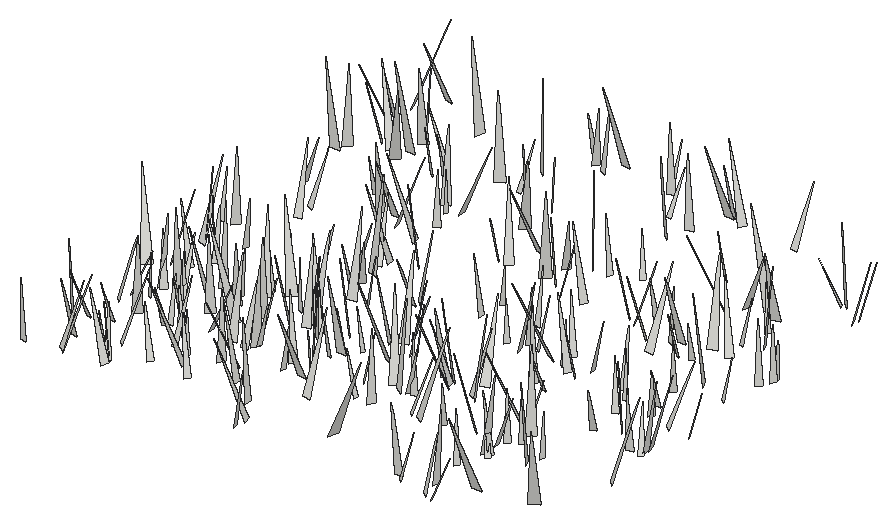
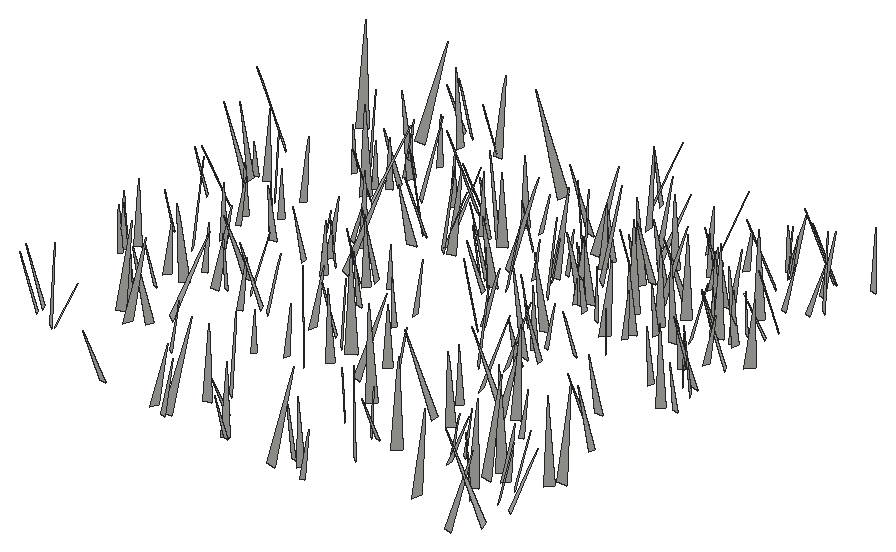
# SketchUp Ruby script. Lengths in inches.
U = 1.inch
M = Sketchup.active_model
def pt(a) = Geom::Point3d.new(a.map { |v| v * U })
def face(e, loops, mat)
  f = e.add_face(loops[0].map { |a| pt(a) })
  loops[1..].each { |l| e.add_face(l.map { |a| pt(a) }).erase! }
  f.material = f.back_material = mat if mat
  f
end
# faces: each face lists its corners as indices into pts; further lists are holes
def faces(e, pts, list, mat = nil) = list.each { |f| face(e, (f[0].is_a?(Array) ? f : [f]).map { |l| l.map { |i| pts[i] } }, mat) }
# xy, xz, yz: faces in a plane at the given z, y or x. An outline is a flat list of corners, or four numbers for a rectangle; further outlines are holes
def ring(l) = l.size == 4 ? [[l[0], l[1]], [l[2], l[1]], [l[2], l[3]], [l[0], l[3]]] : l.each_slice(2).to_a
def flat(e, list, mat, &to3) = list.each { |f| face(e, (f[0].is_a?(Array) ? f : [f]).map { |l| ring(l).map { |u, v| to3.(u, v) } }, mat) }
def xy(e, z, list, mat = nil) = flat(e, list, mat) { |x, y| [x, y, z] }
def xz(e, y, list, mat = nil) = flat(e, list, mat) { |x, z| [x, y, z] }
def yz(e, x, list, mat = nil) = flat(e, list, mat) { |y, z| [x, y, z] }
def lines(e, pts, list) = list.each { |a, b| e.add_line(pt(pts[a]), pt(pts[b])) }
# prism: a flat outline (further loops are holes) pulled along v
def prism(e, loops, v, mat = nil)
  f = face(e, loops, mat); d = Geom::Vector3d.new(v.map { |x| x * U })
  f.pushpull(f.normal.samedirection?(d) ? d.length : -d.length)
end
def box(e, o, s, mat = nil) = prism(e, [[o, [o[0] + s[0], o[1], o[2]], [o[0] + s[0], o[1] + s[1], o[2]], [o[0], o[1] + s[1], o[2]]]], [0, 0, s[2]], mat)
def at(x, y, z, deg = 0) = Geom::Transformation.translation(pt([x, y, z])) * Geom::Transformation.rotation(ORIGIN, Z_AXIS, deg.degrees)
def axes(o, x, y, z) = Geom::Transformation.new([*x, 0, *y, 0, *z, 0, *pt(o).to_a, 1])
def part(name) = M.definitions.add(name)
# library, detail: a bought-in or finely detailed component or shape, given as its bounding box
def library(name, o, s) = part(name).tap { |d| box(d.entities, o, s) }
def detail(e, o, s) = box(e.add_group.entities, o, s)
def put(e, d, t, mat = nil) = e.add_instance(d, t).tap { |i| i.material = mat if mat }
def group(e, t, mat = nil) = e.add_group.tap { |g| g.transformation = t; g.material = mat if mat }.entities
root = M.entities
c1 = part("fur_instance\#9")
p = [[0.8125,0,1.79],[0.67,-0.02,1.48],[0,-0.11,0],[0,0.11,0]]
faces(c1.entities,p,[[0,1,2,3]])
put(root,c1,axes([495.33,166.6,-21.66],[4.4988,1.24272,1.44893],[1.33102,-4.70119,-0.10058],[-1.36826,-0.48722,4.6662]))
put(root,c1,axes([455.36,167.15,-21.66],[1.09401,4.63876,2.44173],[5.21296,-1.22556,-0.00737],[-0.55243,-2.37843,4.76601]))
put(root,c1,axes([531.0625,167.53,-21.66],[3.86213,1.08614,0.2172],[1.09096,-3.86634,-0.0646],[-0.19154,-0.12107,4.01143]))
put(root,c1,axes([495.47,169.01,-21.66],[-6.50715,-2.26194,0.29712],[-2.26712,6.51165,-0.07913],[0.25462,0.17236,6.88863]))
put(root,c1,axes([529.4375,167.89,-21.66],[2.64561,4.33348,1.24236],[4.47199,-2.70465,-0.08904],[-0.56902,-1.10798,5.07645]))
put(root,c1,axes([522.83,170.07,-21.66],[0.27233,-6.25887,1.87066],[-6.53155,-0.29195,-0.02597],[-0.1084,1.8677,6.26474]))
put(root,c1,axes([469.08,168.99,-21.66],[-5.48361,2.04542,0.49712],[2.0602,5.49974,0.09665],[0.43181,-0.2646,5.85187]))
put(root,c1,axes([524,169,-21.66],[2.95956,2.83712,0.75066],[2.89518,-2.997,-0.08741],[-0.48027,-0.58351,4.09885]))
put(root,c1,axes([461.68,168.53,-21.66],[4.96936,4.425,0.65774],[4.44372,-4.99597,0.03757],[-0.51632,-0.4092,6.65385]))
put(root,c1,axes([461.31,168.68,-21.66],[3.13584,4.70476,0.63652],[4.72939,-3.16238,0.0748],[-0.41563,-0.48786,5.65355]))
put(root,c1,axes([534.39,173.77,-21.66],[-0.28609,-7.90952,0.17476],[-7.91116,0.28452,-0.07401],[-0.06767,0.17732,7.91434]))
put(root,c1,axes([468.52,170.24,-21.66],[-1.71851,4.03919,1.0736],[4.16688,1.74577,0.10182],[0.32374,-1.02868,4.3884]))
put(root,c1,axes([467.48,171.24,-21.66],[-3.40834,-0.81843,0.94444],[-0.85751,3.5273,-0.03792],[0.90911,0.25869,3.50503]))
put(root,c1,axes([528.77,171.32,-21.66],[6.1687,-0.67373,2.21616],[-0.70194,-6.55164,-0.0379],[-2.20738,0.2006,6.20527]))
put(root,c1,axes([467.7,171.68,-21.66],[-3.21218,-2.63282,1.4726],[-2.81239,3.39173,-0.07071],[1.09119,0.99138,4.15269]))
put(root,c1,axes([460.17,173,-21.66],[-1.26664,-5.03308,1.07763],[-5.14261,1.28411,-0.04714],[0.2163,1.05675,5.1898]))
put(root,c1,axes([507.95,173.49,-21.66],[8.10386,-2.02713,0.06413],[-2.02706,-8.10412,-0.01624],[-0.06615,-0.00019,8.35354]))
put(root,c1,axes([492.31,173.19,-21.66],[-6.58404,0.20466,2.39247],[0.20033,7.00521,-0.04793],[2.39284,-0.02336,6.58705]))
put(root,c1,axes([543.59,175.66,-21.66],[4.25947,-6.86655,0.67935],[-6.89421,-4.26807,0.08653],[-0.2843,0.62304,8.07992]))
put(root,c1,axes([481,173.25,-21.66],[-3.95377,2.90545,0.68572],[2.92437,3.99824,-0.07937],[0.59996,-0.34142,4.90588]))
put(root,c1,axes([473.61,173.95,-21.66],[-3.58743,2.64736,0.43412],[2.66538,3.59954,0.07504],[0.30449,-0.3184,4.45786]))
put(root,c1,axes([477.97,176.12,-21.66],[-6.75441,-2.93713,0.31923],[-2.94167,6.75982,-0.04619],[0.27431,0.1697,7.36523]))
put(root,c1,axes([457.1875,176.5,-21.66],[-4.34525,-4.69158,2.51984],[-5.05188,4.66036,-0.03462],[1.68493,1.87398,6.3946]))
put(root,c1,axes([487.51,176.7,-21.66],[-6.3571,-0.05635,1.63328],[-0.03082,6.56286,0.10646],[1.63396,-0.09544,6.35645]))
put(root,c1,axes([467.11,175.3,-21.66],[4.12664,4.96749,0.53315],[4.97839,-4.14664,0.10195],[-0.41933,-0.34468,6.45715]))
put(root,c1,axes([458.4375,178.59,-21.66],[-1.93771,-4.14246,0.35212],[-4.15628,1.93921,-0.05843],[0.0961,0.34375,4.57288]))
put(root,c1,axes([527.59,177.65,-21.66],[3.42061,-2.16163,2.16053],[-2.46149,-3.8706,0.02453],[-1.81151,1.17767,4.04631]))
put(root,c1,axes([461.96,179.78,-21.66],[-0.71572,-3.67555,0.46048],[-3.70429,0.70984,-0.09154],[-0.00255,0.46948,3.74347]))
put(root,c1,axes([476.59,178.63,-21.66],[-1.48065,3.15767,1.46809],[3.42197,1.61497,-0.02236],[0.64523,-1.31889,3.48751]))
put(root,c1,axes([484.46,180.79,-21.66],[-3.64802,-5.0358,0.07825],[-5.03596,3.64854,0.02575],[0.06676,0.04827,6.21825]))
put(root,c1,axes([481.78,180.14,-21.66],[5.0258,-2.8928,2.35137],[-3.11716,-5.42578,-0.01254],[-2.04464,1.16127,5.79886]))
put(root,c1,axes([473.82,179.25,-21.66],[1.01663,5.56132,0.68679],[5.60282,-1.02017,-0.03274],[-0.09106,-0.68151,5.65338]))
put(root,c1,axes([493.64,183.99,-21.66],[-0.44109,-6.89492,0.21564],[-6.89758,0.44393,0.08524],[0.09888,0.20974,6.90849]))
put(root,c1,axes([498.125,179.53,-21.66],[1.00933,7.00307,0.82634],[7.04916,-1.02422,0.06983],[-0.18746,-0.80782,7.07509]))
put(root,c1,axes([468.7,183.46,-21.66],[0.77798,-4.23548,0.16889],[-4.23878,-0.77834,0.00619],[-0.02442,0.16723,4.30633]))
put(root,c1,axes([474.21,181.35,-21.66],[-3.97928,1.73175,0.54979],[1.73454,4.01483,-0.09183],[0.54094,-0.13447,4.3388]))
put(root,c1,axes([496.54,182.74,-21.66],[-3.07228,-3.20464,1.70758],[-3.41257,3.31254,0.07678],[1.24093,1.17551,4.43878]))
put(root,c1,axes([528.55,183.05,-21.66],[6.63487,-1.65212,1.91106],[-1.73662,-6.8834,0.0785],[-1.83462,0.54083,6.83702]))
put(root,c1,axes([529.74,182.93,-21.66],[-4.97089,0.8761,1.32855],[0.91857,5.13772,0.0489],[1.29955,-0.28038,5.04727]))
put(root,c1,axes([463.19,183.9375,-21.66],[4.72126,-4.87179,1.88096],[-5.03873,-4.91595,-0.08523],[-1.37242,1.28908,6.78361]))
put(root,c1,axes([529.72,182.17,-21.66],[-3.26703,2.9675,0.38966],[2.97957,3.27925,0.00816],[0.28293,-0.26806,4.41355]))
put(root,c1,axes([490.36,183.92,-21.66],[3.76138,-1.24538,0.93866],[-1.27843,-3.86595,-0.00634],[-0.89313,0.28885,3.96218]))
put(root,c1,axes([535.25,184.36,-21.66],[-5.46396,-3.21591,2.3792],[-3.43589,5.83542,-0.00311],[2.04873,1.20967,6.3401]))
put(root,c1,axes([503.76,183.97,-21.66],[-3.79892,0.58903,0.61511],[0.5899,3.84804,-0.04166],[0.61427,-0.05255,3.84409]))
put(root,c1,axes([506.5,184.14,-21.66],[-5.0872,2.66073,2.45988],[2.85923,5.55214,-0.09239],[2.22604,-1.05084,5.74025]))
put(root,c1,axes([469.13,184.15,-21.66],[-0.34348,3.88251,1.09091],[4.02925,0.37671,-0.07204],[0.17064,-1.07988,3.89701]))
put(root,c1,axes([518.67,185.72,-21.66],[2.48728,-3.44318,0.65298],[-3.47724,-2.52444,-0.0662],[-0.43662,0.49004,4.24707]))
put(root,c1,axes([470.12,185.4,-21.66],[3.33409,-2.8819,1.80128],[-3.12207,-3.59416,0.02846],[-1.34262,1.20116,4.40689]))
put(root,c1,axes([469.6,186.15,-21.66],[-0.47471,-3.8388,0.84095],[-3.92781,0.49062,0.02236],[0.12592,0.83177,3.86797]))
put(root,c1,axes([528.55,185.78,-21.66],[4.6292,0.17151,0.50537],[0.17521,-4.6565,-0.02456],[-0.5041,-0.0434,4.63231]))
put(root,c1,axes([523.57,187.14,-21.66],[-4.39451,-5.32367,1.29551],[-5.40377,4.48556,0.10243],[0.905,0.93264,6.90237]))
put(root,c1,axes([458.69,185.05,-21.66],[3.76051,3.97563,0.83952],[4.01253,-3.81366,0.08642],[-0.64034,-0.54974,5.47171]))
put(root,c1,axes([513.06,185.26,-21.66],[3.32598,3.77438,0.4675],[3.78797,-3.34308,0.04133],[-0.34022,-0.32329,5.03054]))
put(root,c1,axes([474.84,186.57,-21.66],[4.99939,-0.31235,0.02616],[-0.31267,-4.999,0.06629],[-0.02197,0.06779,5.0087]))
put(root,c1,axes([482.875,186.75,-21.66],[-5.61419,2.77509,3.47904],[3.15086,6.4338,-0.04739],[3.14276,-1.49299,6.26243]))
put(root,c1,axes([490.25,186.29,-21.66],[-4.38445,3.57185,1.79964],[3.76738,4.58485,0.07863],[1.34299,-1.20052,5.65467]))
put(root,c1,axes([514.83,184.77,-21.66],[4.48947,6.23838,0.89691],[6.27438,-4.52789,0.08708],[-0.59503,-0.67674,7.68539]))
put(root,c1,axes([536.15,186.82,-21.66],[-3.33469,1.40616,1.82105],[1.56398,3.73727,-0.02186],[1.68745,-0.685,3.61897]))
put(root,c1,axes([482.02,185.29,-21.66],[0.04484,6.03011,0.93276],[6.10111,-0.02998,-0.09948],[0.09373,-0.93336,6.02946]))
put(root,c1,axes([483.18,187.33,-21.66],[3.78435,-1.32179,0.68035],[-1.35222,-3.83372,0.07338],[-0.61764,0.29457,4.00787]))
put(root,c1,axes([479.26,185.82,-21.66],[-0.62472,6.74476,1.37593],[6.88336,0.62526,0.06028],[0.06565,-1.37569,6.77336]))
put(root,c1,axes([529.15,187.35,-21.66],[1.67153,-3.68103,1.97281],[-4.08391,-1.88531,-0.05752],[-0.87388,1.76964,4.04237]))
put(root,c1,axes([531,188.56,-21.66],[1.90593,-3.10212,1.28599],[-3.27722,-2.04084,-0.06594],[-0.73267,1.05893,3.64024]))
put(root,c1,axes([458.91,187.9375,-21.66],[3.47844,1.93474,0.04271],[1.93521,-3.47755,-0.07868],[0.00093,-0.08952,3.97952]))
put(root,c1,axes([487.76,189.89,-21.66],[4.25123,5.18566,4.75994],[6.35301,-5.22113,0.01405],[-3.03108,-3.67013,6.70551]))
put(root,c1,axes([461.67,188.7,-21.66],[1.95949,2.80373,1.45551],[3.04239,-2.136,0.01872],[-0.85045,-1.18135,3.42055]))
put(root,c1,axes([548.44,187.37,-21.66],[5.3088,5.05785,1.00754],[5.10033,-5.36326,0.04959],[-0.76398,-0.65873,7.33231]))
put(root,c1,axes([501.71,188.35,-21.66],[3.13745,2.7412,0.96065],[2.81213,-3.22064,0.00574],[-0.7273,-0.62763,4.16626]))
put(root,c1,axes([482.64,188.22,-21.66],[3.62084,3.81527,1.03017],[3.87963,-3.69771,0.05854],[-0.75237,-0.70613,5.25959]))
put(root,c1,axes([508.8125,189.93,-21.66],[3.98619,-2.41358,0.43201],[-2.42835,-4.00018,0.05811],[-0.33929,0.27366,4.65958]))
put(root,c1,axes([509.96,189.74,-21.66],[-0.91503,4.79321,2.31879],[5.31141,0.98733,0.05504],[0.37492,-2.28894,4.87946]))
put(root,c1,axes([507.33,189.52,-21.66],[3.62939,6.32437,2.66269],[6.74766,-3.83695,-0.08396],[-1.24771,-2.35377,7.2913]))
put(root,c1,axes([471.43,190.52,-21.66],[4.24659,-4.94069,2.32668],[-5.22174,-4.53655,-0.10277],[-1.59916,1.69313,6.51409]))
put(root,c1,axes([528.84,191.89,-21.66],[-5.75391,-4.14909,0.07824],[-4.14913,5.75437,0.02082],[0.07564,0.02888,7.0938]))
put(root,c1,axes([491.06,189.95,-21.66],[5.9616,4.7587,3.0284],[5.08757,-6.43918,0.10304],[-2.43578,-1.80245,7.62727]))
put(root,c1,axes([476.54,190.26,-21.66],[-8.26176,0.40654,0.83522],[0.41692,8.30295,0.08258],[0.83009,-0.12394,8.27135]))
put(root,c1,axes([493.09,191.18,-21.66],[-1.22069,-3.41408,1.05948],[-3.55821,1.26785,-0.01408],[0.34288,1.00256,3.62571]))
put(root,c1,axes([530.64,190.95,-21.66],[5.17413,-4.7343,3.23528],[-5.24163,-5.67192,0.08293],[-2.32507,2.25121,7.01272]))
put(root,c1,axes([464.33,192.09,-21.66],[2.05152,-6.96349,2.48946],[-7.36809,-2.14532,0.07104],[-0.63146,2.40909,7.25905]))
put(root,c1,axes([493.94,192.87,-21.66],[-0.46017,-7.01963,1.64197],[-7.20868,0.46604,-0.02793],[0.07879,1.64032,7.03464]))
put(root,c1,axes([465.36,192.04,-21.66],[2.21811,-2.97156,1.30139],[-3.14682,-2.35396,-0.01147],[-0.78819,1.03561,3.7081]))
put(root,c1,axes([505.71,190.49,-21.66],[-4.53452,6.13099,1.20513],[6.2123,4.58336,0.05748],[0.66981,-1.00349,7.62546]))
put(root,c1,axes([460.99,192.22,-21.66],[5.93404,-1.49093,1.99542],[-1.59561,-6.23409,0.08712],[-1.91274,0.57506,6.11785]))
put(root,c1,axes([461.8,191.83,-21.66],[2.76185,-3.07557,2.49035],[-3.57907,-3.23702,-0.02845],[-1.68858,1.83068,4.13354]))
put(root,c1,axes([529.53,191.36,-21.66],[3.18185,3.17768,0.5905],[3.1987,-3.21478,0.06397],[-0.46337,-0.37158,4.49642]))
put(root,c1,axes([512.22,194.74,-21.66],[-4.64993,-4.92524,0.42817],[-4.93518,4.6591,-0.00251],[0.29211,0.31306,6.77347]))
put(root,c1,axes([465.56,191.13,-21.66],[-0.62554,4.99616,0.12365],[4.99768,0.62512,0.02455],[-0.009,-0.12574,5.03511]))
put(root,c1,axes([500.61,195.39,-21.66],[-3.23676,-6.95107,0.75182],[-6.9834,3.25434,0.02332],[0.33861,0.67166,7.66769]))
put(root,c1,axes([478.29,194.04,-21.66],[5.05478,-5.09898,2.04992],[-5.28407,-5.27475,-0.09077],[-1.51011,1.38923,7.17929]))
put(root,c1,axes([493.68,193.79,-21.66],[-3.08604,-1.58363,1.00431],[-1.62158,3.22493,0.10239],[0.94181,0.36349,3.46714]))
put(root,c1,axes([473.125,194.6,-21.66],[3.25628,-4.96201,1.27437],[-5.08219,-3.31911,0.06246],[-0.64574,1.10043,5.93473]))
put(root,c1,axes([488.24,194.28,-21.66],[2.1369,3.02619,1.55246],[3.28055,-2.31782,0.00255],[-0.89775,-1.26656,3.70461]))
put(root,c1,axes([466.89,195.31,-21.66],[-4.90354,-1.85753,0.89414],[-1.8937,4.97041,-0.05944],[0.81474,0.37312,5.24324]))
put(root,c1,axes([517.3,194.57,-21.66],[-4.33935,-4.28478,3.74469],[-5.00881,5.11096,0.04388],[2.70071,2.59437,6.09815]))
put(root,c1,axes([496.04,195.15,-21.66],[-3.46887,0.5768,0.94943],[0.60796,3.5911,0.03958],[0.92978,-0.19616,3.51628]))
put(root,c1,axes([512.12,195.63,-21.66],[-5.21279,-1.15752,0.50027],[-1.17064,5.23306,-0.0898],[0.46875,0.19648,5.33901]))
put(root,c1,axes([510.08,196.88,-21.66],[1.37866,-6.43403,1.32521],[-6.55871,-1.42426,-0.09169],[-0.36909,1.27608,6.57944]))
put(root,c1,axes([544.63,196.61,-21.66],[1.69924,-5.28596,1.58911],[-5.50046,-1.7602,0.02657],[-0.46001,1.5213,5.5523]))
put(root,c1,axes([511.7,196.83,-21.66],[-4.72321,-4.87597,2.05821],[-5.0831,4.94763,0.05633],[1.47426,1.43735,6.78828]))
put(root,c1,axes([536.71,198.04,-21.66],[2.00782,-4.43373,0.05819],[-4.43409,-2.00742,0.0429],[0.01508,0.0707,4.86698]))
put(root,c1,axes([516.52,194.86,-21.66],[2.68207,4.86571,0.6841],[4.89534,-2.71316,0.10499],[-0.42283,-0.54794,5.55496]))
put(root,c1,axes([487.84,195.44,-21.66],[-3.61656,3.24074,0.55892],[3.26072,3.64166,-0.01623],[0.42715,-0.36083,4.85609]))
put(root,c1,axes([471.99,196.95,-21.66],[-3.43259,1.11019,2.13702],[1.24058,4.00441,-0.08763],[2.06406,-0.56053,3.60659]))
put(root,c1,axes([485.18,195.75,-21.66],[-1.64071,6.20292,1.41522],[6.35653,1.66047,0.09149],[0.27128,-1.39198,6.41559]))
put(root,c1,axes([468.6,197.09,-21.66],[-0.16128,6.84934,2.86842],[7.42417,0.20732,-0.07764],[0.15166,-2.86546,6.8508]))
put(root,c1,axes([491.39,197.9,-21.66],[-4.35453,-4.53446,2.05004],[-4.74623,4.60317,0.10013],[1.49574,1.4055,6.28595]))
put(root,c1,axes([546.71,196.46,-21.66],[-2.11834,3.44874,0.2067],[3.45458,2.11778,0.0692],[0.04913,-0.21236,4.04678]))
put(root,c1,axes([546.7,197.61,-21.66],[6.13024,0.22864,1.74835],[0.20896,-6.37456,0.10097],[-1.75081,0.03976,6.13367]))
put(root,c1,axes([455.26,196.07,-21.66],[-5.44191,5.3364,0.6963],[5.36336,5.45938,0.07682],[0.44311,-0.54257,7.6214]))
put(root,c1,axes([484.33,198.16,-21.66],[5.43956,-0.0104,1.6458],[0.01524,-5.68242,-0.08629],[-1.64576,-0.087,5.43889]))
put(root,c1,axes([486.57,196.85,-21.66],[-5.17368,4.83178,0.63052],[4.85594,5.1888,0.08232],[0.40437,-0.49072,7.07858]))
put(root,c1,axes([485.625,197.01,-21.66],[0.08321,7.29137,1.2347],[7.39423,-0.10178,0.10277],[-0.11831,-1.23331,7.29112]))
put(root,c1,axes([481.32,199.07,-21.66],[-1.7362,-3.80786,1.79903],[-4.13168,1.91701,0.07019],[0.81577,1.60498,4.18441]))
put(root,c1,axes([546.71,198.8,-21.66],[6.30339,2.19635,1.13005],[2.22882,-6.39265,-0.00763],[-1.06457,-0.37914,6.67507]))
put(root,c1,axes([457.78,198.58,-21.66],[5.69643,3.12279,1.00252],[3.16084,-5.76326,-0.00802],[-0.87518,-0.48903,6.49623]))
put(root,c1,axes([497.28,199.88,-21.66],[-4.91949,-2.25789,1.34677],[-2.33985,5.06309,-0.05864],[1.19873,0.61667,5.41258]))
put(root,c1,axes([502.79,199.33,-21.66],[3.09566,2.75124,1.27433],[2.88928,-3.22895,-0.04754],[-0.91941,-0.88367,4.14127]))
put(root,c1,axes([501.86,199.05,-21.66],[5.547,2.87669,1.51326],[2.93945,-5.71712,0.09337],[-1.38744,-0.61131,6.24786]))
put(root,c1,axes([460.85,199.11,-21.66],[-4.64621,2.31988,0.55706],[2.32982,4.67441,-0.03457],[0.51391,-0.21773,5.19306]))
put(root,c1,axes([540.16,200.19,-21.66],[-4.40906,-3.22075,2.19411],[-3.50304,4.72714,-0.10035],[1.70765,1.38134,5.45921]))
put(root,c1,axes([474.79,199.125,-21.66],[-3.82919,5.78151,1.38736],[5.88668,3.91838,-0.08139],[0.83523,-1.11076,6.93412]))
put(root,c1,axes([516.27,198.2,-21.66],[-1.83957,6.80237,0.25254],[6.80704,1.83779,0.08208],[-0.01336,-0.2652,7.04624]))
put(root,c1,axes([474.77,200.69,-21.66],[-3.91308,1.33626,1.31278],[1.41439,4.10109,0.04154],[1.2282,-0.46546,4.13474]))
put(root,c1,axes([523.81,202.68,-21.66],[-1.2303,-3.6424,0.32202],[-3.65502,1.23499,0.00478],[0.10759,0.30356,3.84457]))
put(root,c1,axes([499.16,200.77,-21.66],[-1.91608,6.79372,1.10059],[6.8739,1.94553,-0.04218],[0.33984,-1.04766,7.05863]))
put(root,c1,axes([477.66,201.75,-21.66],[-6.04844,4.67756,1.28768],[4.75602,6.12308,0.0974],[0.95811,-0.86582,7.6455]))
put(root,c1,axes([499.44,202.68,-21.66],[4.10602,0.97464,0.35289],[0.9844,-4.11806,-0.08026],[-0.32469,-0.15985,4.21935]))
put(root,c1,axes([462.84,202.46,-21.66],[-1.62337,4.08317,1.17277],[4.21606,1.70273,-0.09236],[0.52201,-1.05424,4.39307]))
put(root,c1,axes([521.2,203.35,-21.66],[4.8811,-3.48072,2.77846],[-3.79933,-5.40519,-0.09683],[-2.32386,1.52607,5.99426]))
put(root,c1,axes([497.99,203.48,-21.66],[3.13012,3.09581,1.75638],[3.35561,-3.34662,-0.08138],[-1.18695,-1.29717,4.40172]))
put(root,c1,axes([535.99,204,-21.66],[-2.40866,3.6867,1.3913],[3.88066,2.50239,0.08743],[0.68406,-1.21467,4.40293]))
put(root,c1,axes([548.74,205.22,-21.66],[3.66327,1.41122,0.72087],[1.44956,-3.71776,-0.08822],[-0.64027,-0.34277,3.92471]))
put(root,c1,axes([474.44,205.52,-21.66],[2.40837,2.51325,1.53163],[2.71206,-2.66382,0.10655],[-1.14326,-1.0248,3.47927]))
put(root,c1,axes([459.59,206.12,-21.66],[3.22406,2.21993,1.84513],[2.48282,-3.54361,-0.0749],[-1.47248,-1.11442,3.91371]))
put(root,c1,axes([540.6,206.55,-21.66],[2.98723,-2.64764,1.00912],[-2.72025,-3.09017,-0.05514],[-0.79284,0.62671,3.99131]))
put(root,c1,axes([488.04,206.35,-21.66],[3.88099,1.49769,1.22771],[1.56049,-4.04689,0.00388],[-1.14683,-0.43823,4.15995]))
put(root,c1,axes([544.7,205.27,-21.66],[3.10305,4.72146,0.30771],[4.72969,-3.10544,-0.04628],[-0.13026,-0.28259,5.64969]))
put(root,c1,axes([485.26,206.21,-21.66],[-1.01475,7.09695,1.79918],[7.31311,1.06925,-0.09303],[0.3496,-1.76734,7.16853]))
put(root,c1,axes([457.64,205.76,-21.66],[1.8777,6.7714,0.98346],[6.8334,-1.90815,0.09124],[-0.35155,-0.923,7.02632]))
put(root,c1,axes([457.04,207.65,-21.66],[-4.37143,-2.8181,2.86453],[-3.24687,4.97094,-0.06453],[2.3675,1.61389,5.20067]))
put(root,c1,axes([518.65,210.77,-21.66],[-3.40543,-6.99905,0.02732],[-6.9991,3.40539,-0.01642],[-0.00281,0.03175,7.78353]))
put(root,c1,axes([534.7,207.84,-21.66],[-0.32853,3.96848,1.56907],[4.26678,0.33258,0.05223],[0.07349,-1.56822,3.98171]))
put(root,c1,axes([524.65,208.7,-21.66],[-2.53419,-2.69204,0.92744],[-2.77792,2.61003,-0.01451],[0.6248,0.68554,3.69715]))
put(root,c1,axes([539.68,209.39,-21.66],[0.38747,-3.62863,0.53891],[-3.66751,-0.39531,-0.02484],[-0.08219,0.53319,3.64917]))
put(root,c1,axes([463.42,208.81,-21.66],[4.19942,-1.36084,1.21546],[-1.38514,-4.36301,-0.09922],[-1.1877,0.2767,4.41329]))
put(root,c1,axes([493.17,210.67,-21.66],[-1.39577,-4.42794,0.41329],[-4.44248,1.40819,0.08395],[0.20461,0.36877,4.64196]))
put(root,c1,axes([481.99,209.9,-21.66],[-1.43466,-3.23484,0.82707],[-3.31328,1.49057,0.08262],[0.41278,0.72144,3.53774]))
put(root,c1,axes([523.16,208.98,-21.66],[-5.60882,2.54428,1.1021],[2.59069,5.69507,0.03704],[0.9881,-0.48955,6.15881]))
put(root,c1,axes([483.17,211.2,-21.66],[3.21105,-3.45107,0.18225],[-3.45172,-3.21492,-0.06213],[-0.16965,0.09106,4.71348]))
put(root,c1,axes([477.17,209.14,-21.66],[1.79566,3.71313,0.76849],[3.77743,-1.82574,-0.00496],[-0.33004,-0.69403,4.12452]))
put(root,c1,axes([513.52,209.89,-21.66],[5.7925,1.49056,1.34896],[1.52882,-5.93778,-0.00376],[-1.30544,-0.3399,5.9812]))
put(root,c1,axes([510.75,210.29,-21.66],[-2.66914,2.15187,1.53787],[2.38339,2.90414,0.07299],[1.14676,-1.02728,3.42776]))
put(root,c1,axes([521.08,210.0625,-21.66],[-2.34168,-2.41248,1.9117],[-2.76899,2.70012,0.01564],[1.3444,1.35921,3.36204]))
put(root,c1,axes([532.76,209.8125,-21.66],[-0.41482,4.98169,1.32883],[5.15587,0.40286,0.09923],[0.00793,-1.33251,4.99795]))
put(root,c1,axes([513.65,212.1,-21.66],[4.04014,-3.74392,1.13553],[-3.80741,-4.13804,-0.09691],[-0.90002,0.69913,5.50729]))
put(root,c1,axes([525.59,211.6875,-21.66],[4.33952,0.70183,1.00017],[0.70812,-4.45199,0.05164],[-0.99573,-0.10739,4.3956]))
put(root,c1,axes([515.52,211.5625,-21.66],[2.94995,3.39967,1.09614],[3.50655,-3.02709,-0.04841],[-0.68072,-0.86052,4.50085]))
put(root,c1,axes([493.18,211.87,-21.66],[-3.61899,-3.55384,3.43713],[-4.24844,4.41399,0.09065],[2.52873,2.32973,5.07136]))
put(root,c1,axes([458.0625,213.23,-21.66],[-4.38219,4.14776,3.28171],[4.71988,4.98997,-0.0042],[2.38668,-2.25242,6.03386]))
put(root,c1,axes([455.79,212.76,-21.66],[0.08928,4.21713,1.27448],[4.4055,-0.088,-0.01741],[-0.00879,-1.27457,4.21804]))
put(root,c1,axes([538.54,214.15,-21.66],[2.93376,-3.22318,1.07266],[-3.3076,-3.03341,-0.06853],[-0.77414,0.74566,4.35788]))
put(root,c1,axes([480.125,213.73,-21.66],[4.64255,0.07182,0.51653],[0.0806,-4.67045,-0.07504],[-0.51523,-0.08349,4.6425]))
put(root,c1,axes([520.78,213.16,-21.66],[-3.74669,3.50171,1.17991],[3.59906,3.83892,0.03541],[0.8372,-0.8322,5.12819]))
put(root,c1,axes([502.92,214.21,-21.66],[-4.88413,-0.13594,1.40409],[-0.16648,5.08029,-0.08723],[1.4008,0.12978,4.88524]))
put(root,c1,axes([482.7,214.09,-21.66],[2.51079,7.35519,2.45383],[7.71335,-2.63218,-0.00261],[-0.79014,-2.32314,7.77193]))
put(root,c1,axes([546.01,216.47,-21.66],[1.71748,3.11444,0.84575],[3.20742,-1.75327,-0.057],[-0.35706,-0.7688,3.55615]))
put(root,c1,axes([511.01,217.04,-21.66],[0.37459,4.6587,1.44665],[4.87681,-0.39143,-0.00226],[-0.11359,-1.44218,4.67373]))
put(root,c1,axes([482.69,218.3125,-21.66],[-6.22564,-1.43503,0.72375],[-1.44178,6.26598,0.02194],[0.71021,0.14105,6.38885]))
put(root,c1,axes([540.74,218.62,-21.66],[-6.29622,-3.82649,2.40942],[-4.00808,6.63484,0.06324],[2.09347,1.19444,7.36752]))
put(root,c1,axes([503.11,218.79,-21.66],[2.68413,-2.59886,0.79499],[-2.66781,-2.73276,0.07385],[-0.51851,0.60713,3.7354]))
put(root,c1,axes([481.82,216.5625,-21.66],[-1.75814,5.2069,0.13379],[5.20853,1.75836,0.01288],[0.0306,-0.13088,5.4957]))
put(root,c1,axes([486.38,220.1875,-21.66],[-4.69837,-4.55111,2.1601],[-4.81656,4.92378,-0.10244],[1.47629,1.58022,6.5404]))
put(root,c1,axes([463.86,220.32,-21.66],[-1.14776,6.0133,0.84328],[6.0716,1.14805,0.07727],[0.08148,-0.84289,6.12137]))
put(root,c1,axes([532.56,222.75,-21.66],[-2.07432,-2.92088,0.84042],[-3.01146,2.11274,-0.09003],[0.41107,0.73854,3.58137]))
put(root,c1,axes([534.76,223.31,-21.66],[1.50784,-3.41822,0.5063],[-3.4457,-1.52893,-0.06057],[-0.26023,0.4385,3.73552]))
put(root,c1,axes([525.6,224.04,-21.66],[-4.16981,-3.31895,0.85743],[-3.36405,4.22145,-0.01946],[0.65859,0.54939,5.32938]))
put(root,c1,axes([547.18,223.3,-21.66],[2.70237,-4.42657,2.31196],[-4.83243,-2.98105,-0.05917],[-1.25989,1.93941,5.18593]))
put(root,c1,axes([528.59,220.95,-21.66],[0.11708,7.08162,0.20269],[7.08451,-0.11681,-0.01106],[0.00771,-0.20285,7.08258]))
put(root,c1,axes([530.49,226.32,-21.66],[-0.18064,-6.52008,0.8881],[-6.57997,0.17015,-0.08916],[-0.06535,0.89016,6.52198]))
put(root,c1,axes([481.57,225.54,-21.66],[-7.05109,-1.52018,0.70264],[-1.52291,7.08527,0.04653],[0.69669,0.10238,7.21295]))
put(root,c1,axes([548.23,225.35,-21.66],[-3.98978,2.11987,2.03955],[2.3526,4.36264,0.06771],[1.76604,-1.02247,4.51748]))
put(root,c1,axes([463.33,223.76,-21.66],[1.79121,4.66243,0.42191],[4.67903,-1.79759,0.00003],[-0.15134,-0.39383,4.99466]))
put(root,c1,axes([529.24,225.12,-21.66],[1.95895,3.98258,1.69888],[4.26762,-2.09086,-0.01944],[-0.73116,-1.53362,4.43825]))
put(root,c1,axes([548,226.37,-21.66],[2.54214,-2.62214,0.84113],[-2.70032,-2.59808,0.06187],[-0.53981,0.64801,3.65161]))
put(root,c1,axes([519.99,227.26,-21.66],[-3.55733,-3.55392,1.20149],[-3.66341,3.64755,-0.05732],[0.80828,0.89081,5.02808]))
put(root,c1,axes([508.05,226.1875,-21.66],[3.92442,2.27765,0.90763],[2.32456,-4.0011,-0.01041],[-0.77966,-0.46478,4.53747]))
put(root,c1,axes([512.18,226.47,-21.66],[-5.92125,2.00992,1.02968],[2.02644,6.00419,-0.06686],[0.99676,-0.26678,6.25272]))
put(root,c1,axes([521.57,226.55,-21.66],[5.13146,2.31605,0.71954],[2.33013,-5.17519,0.0403],[-0.67253,-0.25897,5.62978]))
put(root,c1,axes([472.16,229.26,-21.66],[3.11086,-6.46121,1.0779],[-6.53922,-3.13316,0.09147],[-0.38422,1.01124,7.17051]))
put(root,c1,axes([474.56,229.64,-21.66],[-0.49515,-5.81147,0.35136],[-5.82208,0.49376,-0.03799],[-0.0081,0.35331,5.8324]))
put(root,c1,axes([503,228.94,-21.66],[4.71718,-6.41333,2.08506],[-6.64537,-4.85367,0.10513],[-1.14777,1.74389,7.96063]))
put(root,c1,axes([505.4,228.24,-21.66],[-3.42106,-4.15596,2.05732],[-4.44833,3.66341,0.00339],[1.31032,1.58608,5.3829]))
put(root,c1,axes([523.79,228.8125,-21.66],[0.76269,-3.95415,0.89534],[-4.04548,-0.80213,-0.09639],[-0.26648,0.86018,4.02588]))
put(root,c1,axes([476.5625,227.5,-21.66],[6.39935,1.66924,0.57136],[1.67346,-6.42366,0.02366],[-0.55885,-0.12123,6.61343]))
put(root,c1,axes([494.44,228.72,-21.66],[-1.9321,-3.03286,0.9193],[-3.13143,1.99261,-0.00754],[0.48737,0.77951,3.596]))
put(root,c1,axes([538.63,227.11,-21.66],[-4.40287,4.25609,0.42122],[4.26988,4.40886,0.08361],[0.24458,-0.35298,6.12311]))
put(root,c1,axes([457.97,229.33,-21.66],[4.67852,-1.7119,0.20248],[-1.71617,-4.68064,0.08066],[-0.16239,0.14538,4.98123]))
put(root,c1,axes([535.25,227.37,-21.66],[-2.63415,6.93544,1.64719],[7.09873,2.71215,-0.06728],[0.64926,-1.51533,7.41852]))
put(root,c1,axes([496.4375,228.63,-21.66],[-4.20959,5.12778,0.85898],[5.1677,4.24809,-0.03415],[0.57165,-0.64206,6.63427]))
put(root,c1,axes([481.34,230.76,-21.66],[2.46407,-3.91283,1.91735],[-4.25122,-2.64198,0.07181],[-0.95581,1.66367,4.6235]))
put(root,c1,axes([503.83,232.76,-21.66],[4.00821,-3.73033,0.31245],[-3.73197,-4.01777,-0.09299],[-0.29215,0.14465,5.47471]))
put(root,c1,axes([497.75,234.18,-21.66],[-1.99035,-6.59495,0.1128],[-6.59501,1.99173,0.07994],[0.10913,0.08488,6.88828]))
put(root,c1,axes([537.77,231,-21.66],[1.92341,3.31368,0.82854],[3.39872,-1.95136,-0.08567],[-0.34002,-0.7604,3.83049]))
put(root,c1,axes([468.19,232.86,-21.66],[0.55845,-3.67703,0.59896],[-3.72525,-0.55803,0.04757],[-0.0423,0.59936,3.71889]))
put(root,c1,axes([540.7,232.79,-21.66],[5.91365,2.78735,2.33328],[2.94924,-6.28377,0.03183],[-2.12497,-0.96423,6.53755]))
put(root,c1,axes([530,237,-21.66],[-4.57477,-6.03245,0.25242],[-6.03633,4.57654,-0.02819],[0.13005,0.21817,7.57088]))
put(root,c1,axes([479.83,234.87,-21.66],[-3.27969,0.65416,1.38528],[0.68941,3.5533,-0.04576],[1.36808,-0.22237,3.34398]))
put(root,c1,axes([506.58,235.58,-21.66],[-5.8561,-4.67693,3.47291],[-5.12361,6.47844,0.0849],[2.77191,2.09401,7.49403]))
put(root,c1,axes([509.93,235.28,-21.66],[-4.33048,1.8912,1.2808],[1.94847,4.49129,-0.04381],[1.19187,-0.47097,4.72523]))
put(root,c1,axes([481.6875,236.18,-21.66],[7.09843,0.26187,0.16049],[0.26265,-7.10014,-0.03187],[-0.15921,-0.03777,7.10319]))
put(root,c1,axes([538.4,236.32,-21.66],[-3.29969,1.99263,1.18367],[2.06312,3.46364,-0.07948],[1.05601,-0.54058,3.85386]))
put(root,c1,axes([491.65,238.38,-21.66],[5.04429,-5.44094,0.7168],[-5.46997,-5.06343,0.05905],[-0.44381,0.56596,7.41924]))
put(root,c1,axes([478.23,236.72,-21.66],[-2.28357,5.70644,2.33564],[6.0895,2.47813,-0.10083],[0.96778,-2.12809,6.14557]))
put(root,c1,axes([514.42,237.35,-21.66],[-2.6188,2.85202,1.01974],[2.95253,2.70449,0.01846],[0.67563,-0.76402,3.87193]))
put(root,c1,axes([537.0625,239.84,-21.66],[1.68994,-6.65431,0.98946],[-6.7239,-1.70391,0.02495],[-0.21912,0.96522,6.8655]))
put(root,c1,axes([455.31,239.73,-21.66],[-0.06707,-7.91469,2.47451],[-8.29222,0.04381,-0.08466],[-0.06773,2.47503,7.91452]))
put(root,c1,axes([531.44,240.21,-21.66],[5.62437,-1.82953,0.08499],[-1.8284,-5.62476,-0.0835],[-0.10665,-0.05312,5.91386]))
put(root,c1,axes([463.97,242.7,-21.66],[5.44226,-5.9088,0.26751],[-5.91243,-5.44486,0.01623],[-0.16928,0.20777,8.03317]))
put(root,c1,axes([456.17,241.5,-21.66],[-4.86484,4.13925,3.64162],[4.78109,5.5858,0.03796],[2.74517,-2.39309,6.38738]))
put(root,c1,axes([471.11,242.48,-21.66],[-2.39364,-3.13142,1.17859],[-3.27618,2.48779,-0.04385],[0.67935,0.9641,3.94124]))
put(root,c1,axes([534.29,241.83,-21.66],[-8.05212,1.79962,1.36323],[1.82873,8.16018,0.02927],[1.32393,-0.32629,8.25072]))
put(root,c1,axes([473.27,242.62,-21.66],[-3.37227,-0.8607,0.92289],[-0.91034,3.4828,-0.07828],[0.87397,0.30665,3.4795]))
put(root,c1,axes([464.56,245.67,-21.66],[-1.19832,-8.06423,2.00487],[-8.30399,1.23724,0.01324],[0.30817,1.98109,8.15276]))
put(root,c1,axes([524,244.62,-21.66],[-2.56443,-3.19615,1.19823],[-3.34404,2.653,-0.08027],[0.6845,0.98675,4.09698]))
put(root,c1,axes([459.35,245.49,-21.66],[-3.89073,-3.2521,0.98713],[-3.3181,3.95947,-0.03367],[0.73538,0.65937,5.07078]))
put(root,c1,axes([491.41,244.86,-21.66],[3.14318,2.78213,1.66083],[2.96777,-3.40061,0.07991],[-1.30037,-1.03624,4.19683]))
put(root,c1,axes([471.76,245.27,-21.66],[-5.15429,0.32159,0.0951],[0.32057,5.15491,-0.05731],[0.09848,0.05128,5.164]))
put(root,c1,axes([461.82,244.46,-21.66],[-5.31881,4.24046,0.31909],[4.24772,5.322,0.07866],[0.20039,-0.26047,6.80184]))
put(root,c1,axes([485.46,246.25,-21.66],[-2.49049,-3.07283,1.62396],[-3.33154,2.67981,-0.03854],[0.99012,1.28779,3.95516]))
put(root,c1,axes([480.12,246.89,-21.66],[4.03772,-5.94106,3.0996],[-6.44975,-4.42725,-0.08397],[-1.8178,2.512,7.18278]))
put(root,c1,axes([546.38,246.15,-21.66],[4.95919,2.18923,1.00137],[2.21006,-5.04934,0.09393],[-0.95452,-0.31696,5.4201]))
put(root,c1,axes([484.25,246.18,-21.66],[1.13394,4.06883,0.24777],[4.07369,-1.14042,0.08414],[-0.14769,-0.216,4.22305]))
put(root,c1,axes([464.42,248.83,-21.66],[2.81734,-6.20209,1.85033],[-6.41792,-2.93797,-0.07572],[-0.83667,1.65211,6.81158]))
put(root,c1,axes([546.32,247.61,-21.66],[4.35259,2.65064,0.87547],[2.69973,-4.40951,-0.0717],[-0.70982,-0.51745,5.09567]))
put(root,c1,axes([541.75,249.27,-21.66],[-3.79405,-1.81524,0.00607],[-1.81515,3.79397,0.03081],[0.01877,-0.02517,4.20582]))
put(root,c1,axes([509.16,249.27,-21.66],[3.99412,4.65299,3.2629],[5.30006,-4.48907,-0.08624],[-2.05092,-2.53923,6.13155]))
put(root,c1,axes([458.83,249.87,-21.66],[-4.42725,-2.60663,1.07476],[-2.66002,4.52485,0.01676],[0.93485,0.53053,5.13759]))
put(root,c1,axes([455.86,251.13,-21.66],[-3.26059,-4.43586,0.10579],[-4.43536,3.26207,0.0775],[0.12511,0.03932,5.50476]))
put(root,c1,axes([542.23,249.74,-21.66],[-4.17203,-5.0841,2.64194],[-5.48144,4.49304,-0.00972],[1.66784,2.04897,6.57676]))
put(root,c1,axes([462.82,251.59,-21.66],[4.34542,2.75412,2.00138],[2.98226,-4.64462,-0.0836],[-1.6422,-1.14703,5.14401]))
put(root,c1,axes([510.52,252.91,-21.66],[-1.61639,5.70202,2.80279],[6.31476,1.76115,0.05886],[0.70173,-2.71416,5.92641]))
put(root,c1,axes([483.26,252.76,-21.66],[4.5767,5.68819,3.18986],[6.17982,-5.02762,0.09872],[-2.08339,-2.41752,7.30013]))
put(root,c1,axes([505.85,254.13,-21.66],[0.74131,3.87524,0.12897],[3.87698,-0.74271,0.03187],[-0.05555,-0.12068,3.94537]))
put(root,c1,axes([469.18,256.02,-21.66],[-7.46216,1.5868,2.36089],[1.65538,7.81249,-0.01867],[2.31332,-0.47194,7.62898]))
put(root,c1,axes([512.72,259.47,-21.66],[-0.43608,-7.58063,0.50958],[-7.59761,0.43802,0.01424],[0.04352,0.50791,7.59315]))
put(root,c1,axes([456.28,256.58,-21.66],[7.55875,3.30018,0.58934],[3.3113,-7.57673,-0.04195],[-0.52327,-0.27436,8.24768]))
put(root,c1,axes([459.4,260.98,-21.66],[-1.29873,-6.18935,0.13887],[-6.18983,1.30082,0.08883],[0.11547,0.11765,6.32352]))
put(root,c1,axes([487.88,259.58,-21.66],[4.42383,-2.92058,1.2942],[-2.99041,-4.56361,-0.07677],[-1.12348,0.64702,5.30039]))
put(root,c1,axes([490.07,258.46,-21.66],[-1.46329,-3.87448,2.4887],[-4.52721,1.6881,-0.03379],[0.84239,2.34204,4.14146]))
put(root,c1,axes([501.87,259.57,-21.66],[2.29625,-5.32789,2.30917],[-5.72704,-2.48806,-0.04565],[-0.95905,2.10109,5.80148]))
put(root,c1,axes([513.0625,260.125,-21.66],[-1.72033,-4.15588,1.09836],[-4.2769,1.77348,0.01157],[0.4311,1.01028,4.49785]))
put(root,c1,axes([515.79,258.65,-21.66],[-6.07575,2.79462,0.62219],[2.80321,6.10345,-0.04049],[0.58225,-0.22305,6.68752]))
put(root,c1,axes([491.56,261.87,-21.66],[-1.16201,-7.65185,1.0654],[-7.72512,1.16361,-0.06847],[0.09162,1.06366,7.73928]))
put(root,c1,axes([526.125,257.77,-21.66],[0.97806,5.36378,0.25201],[5.36787,-0.98334,0.09641],[-0.14015,-0.23057,5.45137]))
put(root,c1,axes([501.68,259.75,-21.66],[0.3484,4.1984,0.59349],[4.23915,-0.35779,0.04247],[-0.09183,-0.58788,4.21262]))
put(root,c1,axes([485.5,262.25,-21.66],[0.8315,-3.67241,0.7269],[-3.73531,-0.86356,-0.09004],[-0.24991,0.6885,3.76429]))
